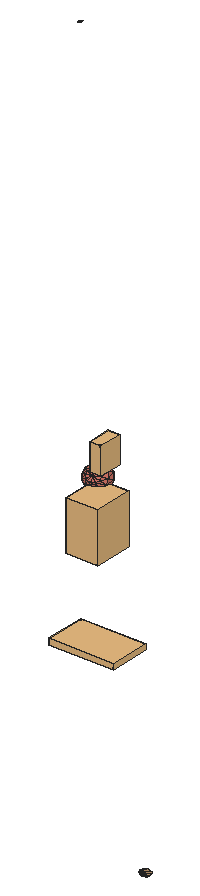
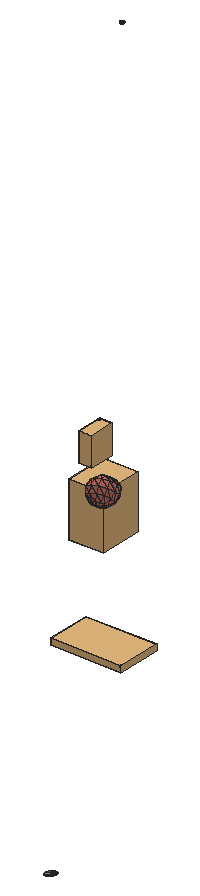
# SketchUp Ruby script. Lengths in inches.
U = 1.inch
M = Sketchup.active_model
def pt(a) = Geom::Point3d.new(a.map { |v| v * U })
def face(e, loops, mat)
  f = e.add_face(loops[0].map { |a| pt(a) })
  loops[1..].each { |l| e.add_face(l.map { |a| pt(a) }).erase! }
  f.material = f.back_material = mat if mat
  f
end
# faces: each face lists its corners as indices into pts; further lists are holes
def faces(e, pts, list, mat = nil) = list.each { |f| face(e, (f[0].is_a?(Array) ? f : [f]).map { |l| l.map { |i| pts[i] } }, mat) }
# xy, xz, yz: faces in a plane at the given z, y or x. An outline is a flat list of corners, or four numbers for a rectangle; further outlines are holes
def ring(l) = l.size == 4 ? [[l[0], l[1]], [l[2], l[1]], [l[2], l[3]], [l[0], l[3]]] : l.each_slice(2).to_a
def flat(e, list, mat, &to3) = list.each { |f| face(e, (f[0].is_a?(Array) ? f : [f]).map { |l| ring(l).map { |u, v| to3.(u, v) } }, mat) }
def xy(e, z, list, mat = nil) = flat(e, list, mat) { |x, y| [x, y, z] }
def xz(e, y, list, mat = nil) = flat(e, list, mat) { |x, z| [x, y, z] }
def yz(e, x, list, mat = nil) = flat(e, list, mat) { |y, z| [x, y, z] }
def lines(e, pts, list) = list.each { |a, b| e.add_line(pt(pts[a]), pt(pts[b])) }
# prism: a flat outline (further loops are holes) pulled along v
def prism(e, loops, v, mat = nil)
  f = face(e, loops, mat); d = Geom::Vector3d.new(v.map { |x| x * U })
  f.pushpull(f.normal.samedirection?(d) ? d.length : -d.length)
end
def box(e, o, s, mat = nil) = prism(e, [[o, [o[0] + s[0], o[1], o[2]], [o[0] + s[0], o[1] + s[1], o[2]], [o[0], o[1] + s[1], o[2]]]], [0, 0, s[2]], mat)
def at(x, y, z, deg = 0) = Geom::Transformation.translation(pt([x, y, z])) * Geom::Transformation.rotation(ORIGIN, Z_AXIS, deg.degrees)
def axes(o, x, y, z) = Geom::Transformation.new([*x, 0, *y, 0, *z, 0, *pt(o).to_a, 1])
def part(name) = M.definitions.add(name)
# library, detail: a bought-in or finely detailed component or shape, given as its bounding box
def library(name, o, s) = part(name).tap { |d| box(d.entities, o, s) }
def detail(e, o, s) = box(e.add_group.entities, o, s)
def put(e, d, t, mat = nil) = e.add_instance(d, t).tap { |i| i.material = mat if mat }
def group(e, t, mat = nil) = e.add_group.tap { |g| g.transformation = t; g.material = mat if mat }.entities
root = M.entities
M.materials.add("green").color = [174, 139, 102]
M.materials.add("vio").color = [206, 114, 100]
c1 = part("3DGeom~213_Defintion")
p = [[-61.03,-133.26,-481.34],[151.11,0,-487.05],[280.8,-170.5625,-375.28],[435.08,-14.45,-265.46],[280.8,-170.5625,-375.28],[-208.41,14.45,-465.11],
  [322.77,133.26,-362.26],[435.08,-14.45,-265.46],[-19.0625,170.56,-468.3125],[-256.82,-230.81,-346.65],[51.28,-280.97,-384.54],[280.8,-170.5625,-375.28],
  [51.28,-280.97,-384.54],[-341.91,-145.53,-337.28],[-256.82,-230.81,-346.65],[-341.91,-145.53,-337.28],[-351.36,122.58,-340.21],[-184.13,295.42,-324.09],
  [175.39,280.97,-346.03],[-424.44,-83.1,-265.17],[-341.91,-145.53,-337.28],[-424.44,-83.1,-265.17],[-191.98,-316.09,-290.76],[51.28,-280.97,-384.54],
  [98.43,-389.1,-200.66],[335.24,-295.42,-162.95],[-256.82,-230.81,-346.65],[51.28,-280.97,-384.54],[-191.98,-316.09,-290.76],[280.8,-170.5625,-375.28],
  [280.8,-170.5625,-375.28],[482.23,-122.58,-81.58],[335.24,-295.42,-162.95],[280.8,-170.5625,-375.28],[435.08,-14.45,-265.46],[322.77,133.26,-362.26],
  [472.78,145.53,-84.51],[175.39,280.97,-346.03],[407.9375,230.81,-140.4],[322.77,133.26,-362.26],[322.77,133.26,-362.26],[-256.82,-230.81,-346.65],
  [-191.98,-316.09,-290.76],[-383.8,-266.51,-119.08],[-341.91,-145.53,-337.28],[-383.8,-266.51,-119.08],[175.39,280.97,-346.03],[322.85,316.09,-131.03],
  [32.44,389.1,-221.13],[32.44,389.1,-221.13],[322.85,316.09,-131.03],[175.39,280.97,-346.03],[-482.31,-60.25,-149.64],[-351.36,122.58,-340.21],
  [-424.44,-83.1,-265.17],[-451.58,162.16,-140.11],[-351.36,122.58,-340.21],[-184.13,295.42,-324.09],[-351.36,122.58,-340.21],[-383.8,-266.51,-119.08],
  [-299.86,341.12,-93.03],[-184.13,295.42,-324.09],[-299.86,341.12,-93.03],[32.44,389.1,-221.13],[-184.13,295.42,-324.09],[-164.76,-378.52,-184.6],
  [-383.8,-266.51,-119.08],[500,83.1,21.65],[-383.8,-266.51,-119.08],[32.44,389.1,-221.13],[240.32,378.52,-58.92],[322.85,316.09,-131.03],
  [-299.86,341.12,-93.03],[-67.78,428.68,-21.03],[32.44,389.1,-221.13],[32.44,389.1,-221.13],[67.78,-428.68,21.03],[299.86,-341.12,93.03],
  [-182.45,-401.37,-56.61],[335.24,-295.42,-162.95],[451.58,-162.16,140.11],[299.86,-341.12,93.03],[335.24,-295.42,-162.95],[-500,-83.1,-21.65],
  [-383.8,-266.51,-119.08],[383.8,266.51,119.08],[-482.23,122.58,81.58],[240.32,378.52,-58.92],[-240.32,-378.52,58.92],[-240.32,-378.52,58.92],
  [-322.85,-316.09,131.03],[-383.8,-266.51,-119.08],[-407.9375,-230.81,140.4],[-383.8,-266.51,-119.08],[-472.78,-145.53,84.51],[-383.8,-266.51,-119.08],
  [-383.8,-266.51,-119.08],[-335.24,295.42,162.95],[-335.24,295.42,162.95],[-299.86,341.12,-93.03],[482.31,60.25,149.64],[182.45,401.37,56.61],
  [383.8,266.51,119.08],[-32.44,-389.1,221.14],[-240.32,-378.52,58.92],[-335.24,295.42,162.95],[-98.43,389.1,200.66],[184.13,-295.42,324.09],
  [184.13,-295.42,324.09],[164.76,378.52,184.6],[383.8,266.51,119.08],[-240.32,-378.52,58.92],[-175.39,-280.97,346.03],[-240.32,-378.52,58.92],
  [-175.39,-280.97,346.03],[-322.85,-316.09,131.03],[-435.08,14.45,265.46],[299.86,-341.12,93.03],[351.36,-122.58,340.21],[184.13,-295.42,324.09],
  [299.86,-341.12,93.03],[351.36,-122.58,340.21],[424.44,83.1,265.17],[341.91,145.53,337.28],[424.44,83.1,265.17],[256.82,230.81,346.65],
  [341.91,145.53,337.28],[191.98,316.09,290.76],[256.82,230.81,346.65],[191.98,316.09,290.76],[383.8,266.51,119.08],[-322.77,-133.26,362.26],
  [-175.39,-280.97,346.03],[424.44,83.1,265.17],[351.36,-122.58,340.21],[424.44,83.1,265.17],[-280.8,170.5625,375.28],[-280.8,170.5625,375.28],
  [-335.24,295.42,162.95],[-51.28,280.97,384.54],[-280.8,170.5625,375.28],[-32.44,-389.1,221.14],[19.0625,-170.56,468.3125],[-175.39,-280.97,346.03],
  [-32.44,-389.1,221.14],[184.13,-295.42,324.09],[351.36,-122.58,340.21],[424.44,83.1,265.17],[341.91,145.53,337.28],[-322.77,-133.26,362.26],
  [-280.8,170.5625,375.28],[-435.08,14.45,265.46],[61.03,133.26,481.34],[191.98,316.09,290.76],[-51.28,280.97,384.54],[256.82,230.81,346.65],
  [191.98,316.09,290.76],[208.41,-14.45,465.11],[-175.39,-280.97,346.03],[-151.11,0,487.05],[-322.77,-133.26,362.26],[-175.39,-280.97,346.03],
  [-322.77,-133.26,362.26],[-280.8,170.5625,375.28],[-51.28,280.97,384.54],[-280.8,170.5625,375.28],[-51.28,280.97,384.54]]
faces(c1.entities,p,[[0,1,2],[1,3,4],[5,1,0],[1,6,7],[5,8,1],[8,6,1],[9,0,10],[0,11,12],
  [13,0,14],[15,5,0],[16,8,5],[16,17,8],[8,18,6],[17,18,8],[19,5,20],[21,16,5],
  [22,23,24],[23,25,24],[26,27,28],[23,29,25],[30,31,32],[33,34,31],[35,36,34],[37,38,39],
  [40,38,36],[41,42,43],[44,41,45],[46,47,38],[17,48,18],[49,50,51],[52,53,54],[52,55,56],
  [55,57,58],[54,44,59],[55,60,61],[62,63,64],[22,24,65],[22,65,66],[34,67,31],[34,36,67],
  [52,54,68],[69,70,71],[72,73,74],[73,70,75],[65,24,76],[24,77,76],[24,25,77],[65,76,78],
  [65,78,66],[79,80,81],[82,31,80],[83,52,84],[83,55,52],[36,38,85],[38,47,85],[83,86,55],
  [86,60,55],[47,87,85],[78,88,66],[89,90,91],[90,92,93],[94,83,95],[92,94,96],[86,97,60],
  [98,73,99],[67,36,85],[31,100,80],[31,67,100],[70,101,102],[73,101,70],[78,76,103],[78,103,104],
  [94,86,83],[105,106,73],[106,101,73],[76,107,103],[76,77,108],[100,67,85],[101,109,110],[106,109,101],
  [111,103,112],[113,114,115],[94,116,86],[116,97,86],[92,116,94],[117,118,119],[120,80,121],[122,100,85],
  [123,124,85],[125,126,85],[127,128,85],[109,129,130],[90,131,92],[90,132,131],[80,133,134],[80,100,135],
  [92,131,116],[116,136,97],[137,106,138],[139,109,106],[139,129,109],[140,139,106],[141,142,143],[144,145,142],
  [146,147,148],[149,150,151],[152,153,154],[152,155,156],[145,157,142],[145,146,157],[146,148,157],[157,148,155],
  [158,159,160],[161,142,159],[157,155,152],[162,159,163],[159,164,165],[159,152,166],[142,157,152],[142,152,159]],"vio")
c2 = library("3DGeom~82_Defintion",[-311.46,-44.07,-500],[622.92,88.14,1000])
c3 = part("3DGeom~83_Defintion")
p = [[-298.62,24.62,-492.72],[-284.8,11.4,-500],[-286.34,4.79,-498.51],[-298.62,24.62,-492.72],[-286.83,18.01,-499.32],[-284.8,11.4,-500],
  [-298.62,24.62,-492.72],[-291.89,22.84,-496.66],[-286.83,18.01,-499.32],[-298.62,24.62,-492.72],[-286.34,4.79,-498.51],[-291.04,-0.05,-495.25],
  [-298.62,24.62,-492.72],[-291.04,-0.05,-495.25],[-297.64,-1.82,-491.09],[-298.62,24.62,-492.72],[-297.64,-1.82,-491.09],[-304.37,-0.05,-487.15],
  [-298.62,24.62,-492.72],[-304.37,-0.05,-487.15],[-309.43,4.79,-484.49],[-298.62,24.62,-492.72],[-309.43,4.79,-484.49],[-311.46,11.4,-483.81],
  [-298.62,24.62,-492.72],[-311.46,11.4,-483.81],[-309.92,18.01,-485.3],[-298.62,24.62,-492.72],[-309.92,18.01,-485.3],[-305.22,22.84,-488.56],
  [307.6,-38.25,479.62],[301.85,-20.79,496.17],[294.12,-44.07,483.45],[307.6,-38.25,479.62],[294.12,-44.07,483.45],[301.3,-42.51,480.25],
  [311.46,-26.61,485.98],[301.85,-20.79,496.17],[307.6,-38.25,479.62],[311.46,-26.61,485.98],[307.6,-38.25,479.62],[311.32,-32.43,481.71],
  [294.12,-44.07,483.45],[301.85,-20.79,496.17],[284.51,-38.25,493.64],[294.12,-44.07,483.45],[284.51,-38.25,493.64],[287.97,-42.51,488.35],
  [301.85,-20.79,496.17],[311.46,-26.61,485.98],[307.99,-22.35,491.27],[284.51,-38.25,493.64],[301.85,-20.79,496.17],[288.37,-26.61,500],
  [284.51,-38.25,493.64],[284.65,-32.43,497.9],[301.85,-20.79,496.17],[294.66,-22.35,499.36]]
faces(c3.entities,p,[[0,1,2],[3,4,5],[6,7,8],[9,10,11],[12,13,14],[15,16,17],[18,19,20],[21,22,23],
  [24,25,26],[27,28,29],[30,31,32],[33,34,35],[36,37,38],[39,40,41],[42,43,44],[45,46,47],
  [48,49,50],[51,52,53],[54,53,55],[56,57,53]],"green")
c4 = library("3DGeom~150_Defintion",[-440.97,-500,-219.09],[881.94,1000,438.17])
c5 = part("3DGeom~151_Defintion")
p = [[-380.69,-485.53,-210.54],[-411.26,-467,-218.1875],[-394.16,-475.51,-219.09],[-380.69,-485.53,-210.54],[-434.74,-476.74,-157.14],[-411.26,-467,-218.1875],
  [-438.29,-462.61,-191.49],[-411.26,-467,-218.1875],[-438.29,-462.61,-191.49],[-427.41,-462.28,-208.09],[-377.14,-499.67,-176.1875],[-434.74,-476.74,-157.14],
  [-380.69,-485.53,-210.54],[-377.14,-499.67,-176.1875],[-380.69,-485.53,-210.54],[-374.46,-494.375,-194.84],[-434.74,-476.74,-157.14],[-440.97,-467.9,-172.84],
  [-438.29,-462.61,-191.49],[-404.17,-495.28,-149.49],[-377.14,-499.67,-176.1875],[-388.02,-500,-159.59],[-404.17,-495.28,-149.49],[-434.74,-476.74,-157.14],
  [-404.17,-495.28,-149.49],[-421.27,-486.76,-148.6],[402.51,492.03,208.37],[431.04,458.58,149.1],[419.28,470.25,140.94],[402.51,492.03,208.37],
  [419.28,470.25,140.94],[406.85,483.28,142.92],[402.51,492.03,208.37],[406.85,483.28,142.92],[397.08,494.17,154.49],[402.51,492.03,208.37],
  [438.98,451.39,165.19],[431.04,458.58,149.1],[402.51,492.03,208.37],[397.08,494.17,154.49],[392.58,500,172.55],[402.51,492.03,208.37],
  [440.97,450.61,184.92],[438.98,451.39,165.19],[402.51,492.03,208.37],[392.58,500,172.55],[394.57,499.22,192.28],[402.51,492.03,208.37],
  [436.48,456.44,202.98],[440.97,450.61,184.92],[402.51,492.03,208.37],[426.7,467.33,214.55],[402.51,492.03,208.37],[414.27,480.36,216.53],
  [426.7,467.33,214.55]]
faces(c5.entities,p,[[0,1,2],[3,4,5],[5,4,6],[7,8,9],[10,11,12],[13,14,15],[16,17,18],[19,20,21],
  [22,11,10],[23,24,25],[26,27,28],[29,30,31],[32,33,34],[35,36,37],[38,39,40],[41,42,43],
  [44,45,46],[47,48,49],[50,51,48],[52,53,54]],"green")
c6 = part("3DGeom~137_Defintion")
p = [[-12.7,499.9,-47.63],[-12.43,498.46,-37.01],[-9.46,500,-49.08],[-9.46,500,-49.08],[-12.43,498.46,-37.01],[-5.93,499.84,-48.71],
  [-9.46,500,-49.08],[-5.93,499.84,-48.71],[-7.64,499.95,-49.12],[-12.7,499.9,-47.63],[-9.46,500,-49.08],[-11.2,499.98,-48.56],
  [-5.93,499.84,-48.71],[-12.43,498.46,-37.01],[-3.15,499.49,-46.71],[-5.93,499.84,-48.71],[-3.15,499.49,-46.71],[-4.41,499.68,-47.89],
  [-13.6875,498.66,-38.1875],[-12.43,498.46,-37.01],[-12.7,499.9,-47.63],[-13.6875,498.66,-38.1875],[-12.7,499.9,-47.63],[-13.9,499.77,-46.38],
  [-3.15,499.49,-46.71],[-12.43,498.46,-37.01],[-1.7,499.01,-43.51],[-3.15,499.49,-46.71],[-1.7,499.01,-43.51],[-2.22,499.26,-45.24],
  [-15.16,499.38,-43.18],[-13.6875,498.66,-38.1875],[-13.9,499.77,-46.38],[-15.16,499.38,-43.18],[-13.9,499.77,-46.38],[-14.73,499.59,-44.87],
  [-1.7,499.01,-43.51],[-12.43,498.46,-37.01],[-2.1,498.55,-40.03],[-1.7,499.01,-43.51],[-2.1,498.55,-40.03],[-1.67,498.77,-41.72],
  [-15.13,499.14,-41.38],[-13.6875,498.66,-38.1875],[-15.16,499.38,-43.18],[-15.13,499.14,-41.38],[-14.61,498.89,-39.66],[-13.6875,498.66,-38.1875],
  [-2.1,498.55,-40.03],[-12.43,498.46,-37.01],[-4.13,498.24,-37.26],[-2.1,498.55,-40.03],[-4.13,498.24,-37.26],[-2.9375,498.375,-38.52],
  [-4.13,498.24,-37.26],[-12.43,498.46,-37.01],[-7.375,498.15,-35.82],[-4.13,498.24,-37.26],[-7.375,498.15,-35.82],[-5.63,498.17,-36.34],
  [-7.375,498.15,-35.82],[-12.43,498.46,-37.01],[-10.9,498.31,-36.19],[-7.375,498.15,-35.82],[-10.9,498.31,-36.19],[-9.2,498.2,-35.78],
  [5.92,-499.89,57.44],[6.49,-499.97,57.1],[7.15,-500,56.9],[5.92,-499.89,57.44],[7.15,-500,56.9],[6.04,-498.77,61.29],
  [7.15,-500,56.9],[8.48,-499.91,57.02],[6.04,-498.77,61.29],[7.15,-500,56.9],[7.84,-499.98,56.88],[8.48,-499.91,57.02],
  [8.48,-499.91,57.02],[9.54,-499.66,57.73],[6.04,-498.77,61.29],[8.48,-499.91,57.02],[9.06,-499.8,57.31],[9.54,-499.66,57.73],
  [5.5625,-498.91,60.87],[5.47,-499.78,57.9],[5.92,-499.89,57.44],[5.5625,-498.91,60.87],[5.92,-499.89,57.44],[6.04,-498.77,61.29],
  [9.54,-499.66,57.73],[10.09,-499.31,58.88],[6.04,-498.77,61.29],[9.54,-499.66,57.73],[9.89,-499.5,58.26],[10.09,-499.31,58.88],
  [5,-499.46,59.0625],[5.16,-499.63,58.45],[5.47,-499.78,57.9],[5,-499.46,59.0625],[5.47,-499.78,57.9],[5.5625,-498.91,60.87],
  [10.09,-499.31,58.88],[9.94,-498.95,60.15],[6.04,-498.77,61.29],[10.09,-499.31,58.88],[10.1,-499.12,59.53],[9.94,-498.95,60.15],
  [5.5625,-498.91,60.87],[5.01,-499.27,59.72],[5,-499.46,59.0625],[5.5625,-498.91,60.87],[5.21,-499.08,60.34],[5.01,-499.27,59.72],
  [9.94,-498.95,60.15],[9.17,-498.68,61.16],[6.04,-498.77,61.29],[9.94,-498.95,60.15],[9.625,-498.8,60.7],[9.17,-498.68,61.16],
  [9.17,-498.68,61.16],[7.95,-498.58,61.7],[6.04,-498.77,61.29],[9.17,-498.68,61.16],[8.61,-498.61,61.5],[7.95,-498.58,61.7],
  [7.95,-498.58,61.7],[6.62,-498.66,61.58],[6.04,-498.77,61.29],[7.95,-498.58,61.7],[7.26,-498.6,61.72],[6.62,-498.66,61.58]]
faces(c6.entities,p,[[0,1,2],[3,4,5],[6,7,8],[9,10,11],[12,13,14],[15,16,17],[18,19,20],[21,22,23],
  [24,25,26],[27,28,29],[30,31,32],[33,34,35],[36,37,38],[39,40,41],[42,43,44],[45,46,47],
  [48,49,50],[51,52,53],[54,55,56],[57,58,59],[60,61,62],[63,64,65],[66,67,68],[69,70,71],
  [72,73,74],[75,76,77],[78,79,80],[81,82,83],[84,85,86],[87,88,89],[90,91,92],[93,94,95],
  [96,97,98],[99,100,101],[102,103,104],[105,106,107],[108,109,110],[111,112,113],[114,115,116],[117,118,119],
  [120,121,122],[123,124,125],[126,127,128],[129,130,131]],"green")
c7 = library("3DGeom~84_Defintion",[-394.11,-500,-321.29],[788.22,1000,642.58])
c8 = part("3DGeom~85_Defintion")
p = [[-385.68,493.0625,-287],[-375.2,479.16,-321.29],[-384.38,476.9375,-316.78],[-385.68,493.0625,-287],[-366.22,483.875,-321.2],[-375.2,479.16,-321.29],
  [-385.68,493.0625,-287],[-359.85,489.82,-316.53],[-366.22,483.875,-321.2],[-385.68,493.0625,-287],[-384.38,476.9375,-316.78],[-391.31,477.81,-308.86],
  [-385.68,493.0625,-287],[-357.79,495.41,-308.52],[-359.85,489.82,-316.53],[-385.68,493.0625,-287],[-391.31,477.81,-308.86],[-394.11,481.53,-299.68],
  [-385.68,493.0625,-287],[-360.59,499.13,-299.34],[-357.79,495.41,-308.52],[-385.68,493.0625,-287],[-394.11,481.53,-299.68],[-392.05,487.11,-291.68],
  [-385.68,493.0625,-287],[-367.52,500,-291.43],[-360.59,499.13,-299.34],[-385.68,493.0625,-287],[-376.7,497.78,-286.91],[-367.52,500,-291.43],
  [382.1,-486.4,280.5],[375.41,-492.22,320.16],[367.13,-497.09,286.29],[382.1,-486.4,280.5],[367.13,-497.09,286.29],[373.98,-492.12,280.77],
  [393.73,-478.62,294.54],[393.73,-478.62,294.54],[382.1,-486.4,280.5],[389.33,-481.46,285.53],[367.13,-497.09,286.29],[363.79,-500,306.12],
  [363.4,-499.97,295.5625],[367.13,-497.09,286.29],[375.41,-492.22,320.16],[363.79,-500,306.12],[390.38,-481.53,314.37],[390.38,-481.53,314.37],
  [393.73,-478.62,294.54],[394.11,-478.65,305.09],[375.41,-492.22,320.16],[368.18,-497.16,315.12],[363.79,-500,306.12],[375.41,-492.22,320.16],
  [390.38,-481.53,314.37],[383.54,-486.5,319.88]]
faces(c8.entities,p,[[0,1,2],[3,4,5],[6,7,8],[9,10,11],[12,13,14],[15,16,17],[18,19,20],[21,22,23],
  [24,25,26],[27,28,29],[30,31,32],[33,34,35],[36,31,30],[37,38,39],[40,41,42],[43,44,45],
  [46,31,36],[47,48,49],[50,51,52],[53,54,55]],"green")
g1 = group(root,at(15.3125,134.49,26.21))
put(g1,c1,axes([-1.84,0.51,8.4],[0,0.00038,0],[0,0,-0.00038],[-0.00038,0,0]),"vio")
g2 = group(root,at(15.3125,134.49,26.21))
put(g2,c2,axes([-1.65,0.26,6.38],[0,0.00095,0],[0,0,-0.00095],[-0.00095,0,0]),"green")
put(g2,c3,axes([-1.65,0.26,6.38],[0,0.00095,0],[0,0,-0.00095],[-0.00095,0,0]),"green")
g3 = group(root,at(15.3125,134.49,26.21))
put(g3,c4,axes([-1.63,0.37,8.85],[0,0.00039,0],[0,0,-0.00039],[-0.00039,0,0]),"green")
put(g3,c5,axes([-1.63,0.37,8.85],[0,0.00039,0],[0,0,-0.00039],[-0.00039,0,0]),"green")
put(root,c6,axes([13.77,135.02,35.07],[0,0.01074,0],[0,0,-0.01074],[-0.01074,0,0]),"green")
g4 = group(root,at(15.3125,134.49,26.21))
put(g4,c7,axes([-1.61,0.21,8.02],[0,0.00073,0],[0,0,-0.00073],[-0.00073,0,0]),"green")
put(g4,c8,axes([-1.61,0.21,8.02],[0,0.00073,0],[0,0,-0.00073],[-0.00073,0,0]),"green")
